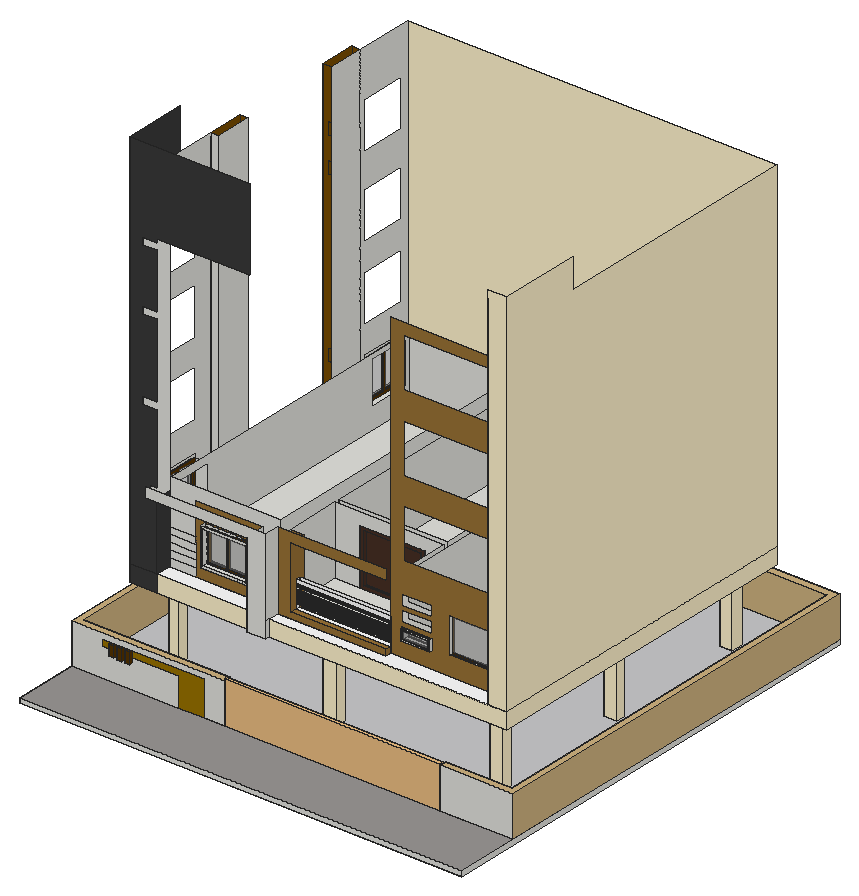
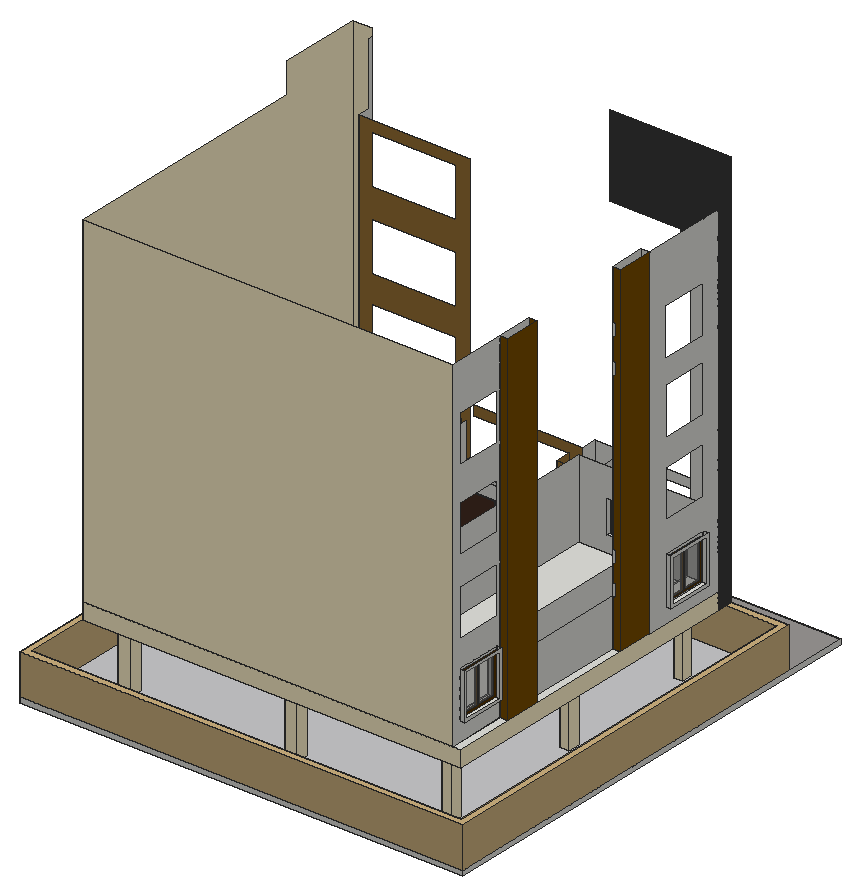
# SketchUp Ruby script. Lengths in inches.
U = 1.inch
M = Sketchup.active_model
def pt(a) = Geom::Point3d.new(a.map { |v| v * U })
def face(e, loops, mat)
  f = e.add_face(loops[0].map { |a| pt(a) })
  loops[1..].each { |l| e.add_face(l.map { |a| pt(a) }).erase! }
  f.material = f.back_material = mat if mat
  f
end
# faces: each face lists its corners as indices into pts; further lists are holes
def faces(e, pts, list, mat = nil) = list.each { |f| face(e, (f[0].is_a?(Array) ? f : [f]).map { |l| l.map { |i| pts[i] } }, mat) }
# xy, xz, yz: faces in a plane at the given z, y or x. An outline is a flat list of corners, or four numbers for a rectangle; further outlines are holes
def ring(l) = l.size == 4 ? [[l[0], l[1]], [l[2], l[1]], [l[2], l[3]], [l[0], l[3]]] : l.each_slice(2).to_a
def flat(e, list, mat, &to3) = list.each { |f| face(e, (f[0].is_a?(Array) ? f : [f]).map { |l| ring(l).map { |u, v| to3.(u, v) } }, mat) }
def xy(e, z, list, mat = nil) = flat(e, list, mat) { |x, y| [x, y, z] }
def xz(e, y, list, mat = nil) = flat(e, list, mat) { |x, z| [x, y, z] }
def yz(e, x, list, mat = nil) = flat(e, list, mat) { |y, z| [x, y, z] }
def lines(e, pts, list) = list.each { |a, b| e.add_line(pt(pts[a]), pt(pts[b])) }
# prism: a flat outline (further loops are holes) pulled along v
def prism(e, loops, v, mat = nil)
  f = face(e, loops, mat); d = Geom::Vector3d.new(v.map { |x| x * U })
  f.pushpull(f.normal.samedirection?(d) ? d.length : -d.length)
end
def box(e, o, s, mat = nil) = prism(e, [[o, [o[0] + s[0], o[1], o[2]], [o[0] + s[0], o[1] + s[1], o[2]], [o[0], o[1] + s[1], o[2]]]], [0, 0, s[2]], mat)
def at(x, y, z, deg = 0) = Geom::Transformation.translation(pt([x, y, z])) * Geom::Transformation.rotation(ORIGIN, Z_AXIS, deg.degrees)
def axes(o, x, y, z) = Geom::Transformation.new([*x, 0, *y, 0, *z, 0, *pt(o).to_a, 1])
def part(name) = M.definitions.add(name)
# library, detail: a bought-in or finely detailed component or shape, given as its bounding box
def library(name, o, s) = part(name).tap { |d| box(d.entities, o, s) }
def detail(e, o, s) = box(e.add_group.entities, o, s)
def put(e, d, t, mat = nil) = e.add_instance(d, t).tap { |i| i.material = mat if mat }
def group(e, t, mat = nil) = e.add_group.tap { |g| g.transformation = t; g.material = mat if mat }.entities
root = M.entities
M.materials.add("[Color C07]").color = [120, 76, 0]
M.materials.add("[Color C08]").color = [85, 51, 0]
M.materials.add("[Color D01]").color = [255, 242, 204]
M.materials.add("[Color D07]").color = [153, 114, 54]
M.materials.add("[Color D07]1").color = [153, 114, 0]
M.materials.add("[Color D08]").color = [95, 67, 39]
M.materials.add("[Color M00]").color = [255, 255, 255]
M.materials.add("[Color M07]").color = [58, 58, 58]
M.materials.add("[Concrete Aggregate Smoke]").color = [154, 150, 148]
M.materials.add("[Polished Concrete New]").color = [200, 200, 203]
M.materials.add("[Stone Sandstone Ashlar Light]").color = [206, 178, 128]
M.materials.add("[Translucent Glass Gray]").color = [128, 128, 128]
M.materials["[Translucent Glass Gray]"].alpha = 0.5
M.materials.add("[Wood Veneer 01]").color = [71, 47, 37]
c1 = library("gate 512k",[0,0,0],[179,6.5,74.5])
c2 = part("Group\#2")
xy(c2.entities,0,[[0,0,105.3125,8.625]],"[Wood Veneer 01]")
xy(c2.entities,6.5,[[6.5,0,98.81,8.625]],"[Wood Veneer 01]")
xy(c2.entities,132.37,[[6.5,0,98.81,8.625]],"[Wood Veneer 01]")
xy(c2.entities,138.875,[[0,0,105.3125,8.625]],"[Wood Veneer 01]")
xz(c2.entities,0,[[[0,0,105.3125,138.875],[6.5,6.5,98.81,132.37]]],"[Wood Veneer 01]")
xz(c2.entities,8.625,[[[0,0,105.3125,138.875],[6.5,6.5,98.81,132.37]],[6.5,6.5,98.81,132.37]],"[Wood Veneer 01]")
yz(c2.entities,0,[[0,0,8.625,138.875]],"[Wood Veneer 01]")
yz(c2.entities,6.5,[[0,6.5,8.625,132.37]],"[Wood Veneer 01]")
yz(c2.entities,98.81,[[0,6.5,8.625,132.37]],"[Wood Veneer 01]")
yz(c2.entities,105.3125,[[0,0,8.625,138.875]],"[Wood Veneer 01]")
c3 = part("Group\#4")
xy(c3.entities,0,[[0,0,0.4375,8.25]],"[Color C08]")
xy(c3.entities,9.875,[[0,0,0.4375,8.25]],"[Color C08]")
xz(c3.entities,0,[[0,0,0.4375,9.875]],"[Color C08]")
xz(c3.entities,0.45,[[0,0.45,0.4375,9.42]],"[Color C08]")
xz(c3.entities,4.05,[[0,0.49,0.4375,9.45]],"[Color C08]")
xz(c3.entities,4.38,[[0,0.49,0.4375,9.45]],"[Color C08]")
xz(c3.entities,7.8,[[0,0.45,0.4375,9.42]],"[Color C08]")
xz(c3.entities,8.25,[[0,0,0.4375,9.875]],"[Color C08]")
yz(c3.entities,0,[[[0,0,8.25,9.875],[0.45,0.45,4.05,0.49,4.05,9.45,0.45,9.42],[7.8,0.45,7.8,9.42,4.38,9.45,4.38,0.49]]],"[Color C08]")
yz(c3.entities,0,[[0.45,0.45,0.45,9.42,4.05,9.45,4.05,0.49],[7.8,0.45,4.38,0.49,4.38,9.45,7.8,9.42]],"[Translucent Glass Gray]")
yz(c3.entities,0.4375,[[[0,0,8.25,9.875],[0.45,0.45,0.45,9.42,4.05,9.45,4.05,0.49],[7.8,0.45,4.38,0.49,4.38,9.45,7.8,9.42]]],"[Color C08]")
p = [[0,4.05,0.49],[0,0.45,0.45],[0.4375,0.45,0.45],[0.4375,4.05,0.49],[0,7.8,0.45],[0,4.38,0.49],
  [0.4375,4.38,0.49],[0.4375,7.8,0.45],[0,0.45,9.42],[0,4.05,9.45],[0.4375,4.05,9.45],[0.4375,0.45,9.42],
  [0,4.38,9.45],[0,7.8,9.42],[0.4375,7.8,9.42],[0.4375,4.38,9.45]]
faces(c3.entities,p,[[0,1,2,3],[4,5,6,7],[8,9,10,11],[12,13,14,15]],"[Color C08]")
c4 = part("Group\#3")
xy(c4.entities,0,[[0,0,69.125,3.25]],"[Color C08]")
xy(c4.entities,1.72,[[1.72,0,67.41,3.25]],"[Color C08]")
xy(c4.entities,48.28,[[1.72,0,67.41,3.25]],"[Color C08]")
xy(c4.entities,50,[[0,0,69.125,3.25]],"[Color C08]")
xz(c4.entities,0,[[[0,0,69.125,50],[1.72,1.72,67.41,48.28]]],"[Color C08]")
xz(c4.entities,0,[[1.72,1.72,67.41,48.28]],"[Translucent Glass Gray]")
xz(c4.entities,3.25,[[[0,0,69.125,50],[1.72,1.72,67.41,48.28]]],"[Color C08]")
yz(c4.entities,0,[[0,0,3.25,50]],"[Color C08]")
yz(c4.entities,1.72,[[0,1.72,3.25,48.28]],"[Color C08]")
yz(c4.entities,67.41,[[0,1.72,3.25,48.28]],"[Color C08]")
yz(c4.entities,69.125,[[0,0,3.25,50]],"[Color C08]")
xy(root,0,[[0,0,780,833.125]])
xy(root,9,[[0,113.125,0,833.125,780,833.125,780,113.125,650.79,113.125,650.79,125.125,768,125.125,768,821.125,12,821.125,12,125.125,270.04,125.125,270.04,113.125],[96,209.125,112.5,227.9375],[367.78,209.125,390.9375,227.9375],[661.375,209.125,684,227.9375],[96,457.125,112.5,477.92],
  [661.375,461.49,684,477.92],[96,716.3125,112.5,737.125],[368.72,716.3125,389.47,737.125],[661.375,716.3125,684,737.125]])
xy(root,9,[[0,0,780,0,780,113.125,650.79,113.125,650.79,125.125,270.04,125.125,270.04,113.125,0,113.125]],"[Concrete Aggregate Smoke]")
xy(root,9,[[[12,125.125,768,821.125],[661.375,716.3125,684,737.125],[367.78,209.125,390.9375,227.9375],[368.72,716.3125,389.47,737.125],[661.375,209.125,684,227.9375],[661.375,461.49,684,477.92],[96,716.3125,112.5,737.125],[96,457.125,112.5,477.92],[96,209.125,112.5,227.9375]]],"[Polished Concrete New]")
xy(root,50.58,[[69.4,108.8125,78.47,113.125],[83.09,108.8125,92.15,113.125],[97.09,108.8125,106.15,113.125]],"[Color C08]")
xy(root,70.7,[[69.4,108.8125,78.47,113.125],[83.09,108.8125,92.15,113.125],[97.09,108.8125,106.15,113.125]],"[Color C08]")
xy(root,81,[[0,113.125,270.04,113.125,270.04,125.125,12,125.125,12,821.125,768,821.125,768,125.125,650.79,125.125,650.79,113.125,780,113.125,780,833.125,0,833.125]],"[Stone Sandstone Ashlar Light]")
xy(root,129,[[261.34,172.6875,295.1875,180.75],[96,209.125,112.5,227.9375],[367.78,209.125,390.9375,227.9375],[661.375,209.125,684,227.9375],[96,457.125,112.5,477.92],
  [661.375,461.49,684,477.92],[96,716.3125,112.5,737.125],[368.72,716.3125,389.47,737.125],[661.375,716.3125,684,737.125]])
xy(root,129,[[48.625,180.75,715.3125,776.25]],"[Color D01]")
xy(root,158,[[75,180.75,95.94,209.375],[681.47,180.75,715.3125,209.375],[295.1875,199.5625,318.6875,227.625],[318.6875,199.5625,486.25,218.375],[48.625,209.375,48.625,360.49,63,360.49,63,776.25,715.3125,776.25,715.3125,209.375,486.25,209.375,486.25,326.375,453.52,326.375,453.52,335.375,486.25,335.375,486.25,764.25,495.25,764.25,495.25,218.375,703.3125,218.375,703.3125,764.25,75,764.25,75,218.375,286.1875,218.375,286.1875,764.25,295.1875,764.25,295.1875,335.375,337.77,335.375,337.77,326.375,295.1875,326.375,295.1875,209.375],
  [75,218.375,286.1875,764.25],[318.6875,218.375,486.25,218.375,486.25,326.375,453.52,326.375,453.52,335.375,337.77,335.375,337.77,326.375,295.1875,326.375,295.1875,227.625,318.6875,227.625],[495.25,218.375,703.3125,764.25],[295.1875,335.375,486.25,764.25],[48.625,360.49,63,423.72],
  [48.625,423.72,63,608.17],[48.625,608.17,63,671.4],[48.625,671.4,63,776.25]])
xy(root,158,[[95.94,180.75,261.34,209.375],[295.1875,180.75,295.1875,199.5625,486.25,199.5625,486.25,209.375,681.47,209.375,681.47,180.75]],"[Color M00]")
xy(root,168.375,[[318.6875,199.5625,486.25,209.375]],"[Color D07]")
xy(root,168.375,[[318.6875,209.375,486.25,218.375]],"[Color M00]")
xy(root,182.15,[[158.4,200.375,241.77,209.375]])
xy(root,185.7,[[39.625,241.8125,48.625,325.0625]])
xy(root,186.15,[[162.4,200.375,237.77,209.375],[162.4,209.375,237.77,218.375]])
xy(root,186.74,[[507.06,205.375,558.75,209.375]])
xy(root,188.74,[[509.06,205.375,556.75,209.375],[509.06,209.375,556.75,218.375]])
xy(root,189.7,[[39.625,245.8125,48.625,321.0625],[48.625,245.8125,75,321.0625]])
xy(root,191.68,[[591.14,209.375,681.47,218.375]])
xy(root,191.73,[[54,679.03,63,761.4]])
xy(root,195.73,[[54,683.03,63,757.4],[63,683.03,75,757.4]])
xy(root,203.99,[[509.06,205.375,556.75,209.375],[509.06,209.375,556.75,218.375]])
xy(root,205.99,[[507.06,205.375,558.75,209.375]])
xy(root,209.5,[[318.6875,209.375,486.25,218.375]],"[Color M00]")
xz(root,0,[[0,0,780,9]])
xz(root,108.8125,[[69.4,50.58,78.47,70.7],[83.09,50.58,92.15,70.7],[97.09,50.58,106.15,70.7]],"[Color C08]")
xz(root,113.125,[[0,9,188.59,9,188.59,58.95,106.15,58.95,106.15,50.58,97.09,50.58,97.09,58.95,92.15,58.95,92.15,50.58,83.09,50.58,83.09,58.95,78.47,58.95,78.47,50.58,69.4,50.58,69.4,58.95,53.21,58.95,53.21,70.7,235.65,70.7,235.65,9,270.04,9,270.04,81,0,81],[650.79,9,780,81]])
xz(root,113.125,[[69.4,50.58,78.47,70.7],[83.09,50.58,92.15,70.7],[97.09,50.58,106.15,70.7]],"[Color C08]")
xz(root,113.125,[[188.59,9,235.65,9,235.65,70.7,106.15,70.7,106.15,58.95,188.59,58.95],[53.21,58.95,69.4,70.7],[78.47,58.95,83.09,70.7],[92.15,58.95,97.09,70.7]],"[Color D07]1")
xz(root,125.125,[[12,9,270.04,81],[650.79,9,768,81]],"[Stone Sandstone Ashlar Light]")
xz(root,172.6875,[[261.34,129,295.1875,129,295.1875,295,83.63,295,83.63,278,261.34,278]])
xz(root,180.75,[[95.94,129,261.34,158],[295.1875,129,715.3125,158],[681.47,158,715.3125,814.1875]],"[Color D01]")
xz(root,180.75,[[48.625,129,95.94,158],[48.625,158,95.94,158,95.94,278,83.63,278,83.63,295,95.94,295,95.94,418.67,70.87,418.67,70.87,431.12,95.94,431.12,95.94,561.36,70.87,561.36,70.87,573.81,95.94,573.81,95.94,670.36,70.87,670.36,70.87,682.81,95.94,682.81,95.94,689,261.34,689,261.34,833,48.625,833]],"[Color M07]")
xz(root,199.5625,[[295.1875,158,486.25,158,486.25,168.375,318.6875,168.375,318.6875,278,486.25,278,486.25,295,295.1875,295]],"[Color D07]")
xz(root,200.375,[[[158.4,182.15,241.77,248.34],[162.4,186.15,237.77,244.34]]])
xz(root,205.375,[[[507.06,186.74,558.75,205.99],[509.06,188.74,556.75,203.99]]])
xz(root,209.125,[[96,9,112.5,129],[367.78,9,390.9375,129],[661.375,9,684,129]],"[Color D01]")
xz(root,209.375,[[48.625,158,95.94,689],[95.94,158,143.14,172.15],[95.94,172.15,143.14,184.34],[[158.4,182.15,241.77,248.34],[162.4,186.15,237.77,244.34]],[95.94,184.34,143.14,196.52],
  [[507.06,186.74,558.75,205.99],[509.06,188.74,556.75,203.99]],[95.94,196.52,143.14,208.71],[95.94,208.71,143.14,220.9]])
xz(root,209.375,[[[143.14,158,261.34,278],[158.4,182.15,241.77,248.34]],[[486.25,158,681.47,158,681.47,191.68,591.14,191.68,591.14,253.18,681.47,253.18,681.47,689,486.25,689],[510.53,312.03,659.59,398.84],[510.53,446.34,659.59,533.16],[510.53,583.28,659.59,670.09],[507.06,240.37,558.75,259.62],[507.06,186.74,558.75,205.99],[507.06,214.49,558.75,233.74]]],"[Color D07]")
xz(root,209.375,[[318.6875,209.5,486.25,216.375]],"[Color M00]")
xz(root,218.375,[[[75,158,286.1875,295],[162.4,186.15,237.77,244.34]],[318.6875,158,486.25,168.375],[[495.25,158,703.3125,278],[591.14,191.68,681.47,253.18],[509.06,188.74,556.75,203.99],[509.06,216.49,556.75,231.74],[509.06,242.37,556.75,257.62]]])
xz(root,218.375,[[318.6875,209.5,486.25,216.375]],"[Color M00]")
xz(root,227.625,[[295.1875,158,318.6875,278]],"[Color D07]")
xz(root,227.9375,[[96,9,112.5,129],[367.78,9,390.9375,129],[661.375,9,684,129]],"[Color D01]")
xz(root,241.8125,[[39.625,185.7,48.625,268.95]])
xz(root,245.8125,[[39.625,189.7,48.625,264.95],[48.625,189.7,75,264.95]])
xz(root,321.0625,[[39.625,189.7,48.625,264.95],[48.625,189.7,75,264.95]])
xz(root,325.0625,[[39.625,185.7,48.625,268.95]])
xz(root,326.375,[[295.1875,158,337.77,158,337.77,256.3125,453.52,256.3125,453.52,158,486.25,158,486.25,278,295.1875,278]])
xz(root,335.375,[[295.1875,158,295.1875,278,486.25,278,486.25,158,453.52,158,453.52,256.3125,337.77,256.3125,337.77,158]])
xz(root,360.49,[[48.625,158,63,761]])
xz(root,423.72,[[48.625,158,48.625,761,63,761,63,673.33,56.4375,673.33,56.4375,651.9375,63,651.9375,63,611.45,56.4375,611.45,56.4375,590.06,63,590.06,63,315.01,56.4375,315.01,56.4375,293.62,63,293.62,63,261.95,56.4375,261.95,56.4375,240.56,63,240.56,63,158]],"[Color C07]")
xz(root,457.125,[[96,9,112.5,129]],"[Color D01]")
xz(root,461.49,[[661.375,9,684,129]],"[Color D01]")
xz(root,477.92,[[96,9,112.5,129],[661.375,9,684,129]],"[Color D01]")
xz(root,608.17,[[48.625,158,63,158,63,240.56,56.4375,240.56,56.4375,261.95,63,261.95,63,293.62,56.4375,293.62,56.4375,315.01,63,315.01,63,590.06,56.4375,590.06,56.4375,611.45,63,611.45,63,651.9375,56.4375,651.9375,56.4375,673.33,63,673.33,63,761,48.625,761]],"[Color C07]")
xz(root,671.4,[[48.625,158,63,761]],"[Color C07]")
xz(root,679.03,[[54,191.73,63,274.1]])
xz(root,683.03,[[54,195.73,63,270.1],[63,195.73,75,270.1]])
xz(root,716.3125,[[96,9,112.5,129],[368.72,9,389.47,129],[661.375,9,684,129]],"[Color D01]")
xz(root,737.125,[[96,9,112.5,129],[368.72,9,389.47,129],[661.375,9,684,129]],"[Color D01]")
xz(root,757.4,[[54,195.73,63,270.1],[63,195.73,75,270.1]])
xz(root,761.4,[[54,191.73,63,274.1]])
xz(root,764.25,[[75,158,286.1875,278],[286.1875,158,295.1875,278],[295.1875,158,486.25,278],[486.25,158,495.25,278],[495.25,158,703.3125,278]])
xz(root,776.25,[[48.625,129,715.3125,158],[63,158,715.3125,761]],"[Color D01]")
xz(root,821.125,[[12,9,768,81]],"[Stone Sandstone Ashlar Light]")
xz(root,833.125,[[0,0,780,9]])
xz(root,833.125,[[0,9,780,81]],"[Stone Sandstone Ashlar Light]")
yz(root,0,[[0,0,833.125,9]])
yz(root,0,[[113.125,9,833.125,81]],"[Stone Sandstone Ashlar Light]")
yz(root,12,[[125.125,9,821.125,81]],"[Stone Sandstone Ashlar Light]")
yz(root,39.625,[[[241.8125,185.7,325.0625,268.95],[245.8125,189.7,321.0625,264.95]]])
yz(root,48.625,[[[209.375,158,360.49,761],[242.5625,577.63,325.8125,660.88],[241.8125,452.07,325.0625,535.32],[241.8125,322.38,325.0625,405.63],[241.8125,185.7,325.0625,268.95]],[[241.8125,185.7,325.0625,268.95],[245.8125,189.7,321.0625,264.95]]])
yz(root,48.625,[[360.49,158,423.72,761],[608.17,158,671.4,761]],"[Color C07]")
yz(root,48.625,[[209.375,129,776.25,158]],"[Color D01]")
yz(root,48.625,[[180.75,129,180.75,833,291.52,833,291.52,761,209.375,761,209.375,129]],"[Color M07]")
yz(root,54,[[[679.03,191.73,761.4,274.1],[683.03,195.73,757.4,270.1]]])
yz(root,63,[[360.49,158,423.72,761],[423.72,158,608.17,240.56],[608.17,158,671.4,761],[[671.4,158,776.25,761],[679.03,595.54,761.4,677.91],[679.03,453.91,761.4,536.29],[679.03,321.73,761.4,404.1],[679.03,191.73,761.4,274.1]],[[679.03,191.73,761.4,274.1],[683.03,195.73,757.4,270.1]]])
yz(root,69.4,[[108.8125,50.58,113.125,70.7]],"[Color C08]")
yz(root,75,[[[218.375,158,764.25,278],[245.8125,189.7,321.0625,264.95],[683.03,195.73,757.4,270.1]]])
yz(root,78.47,[[108.8125,50.58,113.125,70.7]],"[Color C08]")
yz(root,83.09,[[108.8125,50.58,113.125,70.7]],"[Color C08]")
yz(root,92.15,[[108.8125,50.58,113.125,70.7]],"[Color C08]")
yz(root,95.94,[[180.75,158,209.375,278]],"[Color M07]")
yz(root,96,[[209.125,9,227.9375,129],[457.125,9,477.92,129],[716.3125,9,737.125,129]],"[Color D01]")
yz(root,97.09,[[108.8125,50.58,113.125,70.7]],"[Color C08]")
yz(root,106.15,[[108.8125,50.58,113.125,70.7]],"[Color C08]")
yz(root,112.5,[[209.125,9,227.9375,129],[457.125,9,477.92,129],[716.3125,9,737.125,129]],"[Color D01]")
yz(root,158.4,[[200.375,182.15,209.375,248.34]])
yz(root,162.4,[[200.375,186.15,209.375,244.34],[209.375,186.15,218.375,244.34]])
yz(root,237.77,[[200.375,186.15,209.375,244.34],[209.375,186.15,218.375,244.34]])
yz(root,241.77,[[200.375,182.15,209.375,248.34]])
yz(root,261.34,[[172.6875,129,172.6875,278,209.375,278,209.375,158,180.75,158,180.75,129]])
yz(root,270.04,[[113.125,9,125.125,81]],"[Stone Sandstone Ashlar Light]")
yz(root,286.1875,[[218.375,158,764.25,295]])
yz(root,295.1875,[[172.6875,129,180.75,158],[172.6875,158,199.5625,295],[199.5625,158,227.625,278],[227.625,158,326.375,278],[335.375,158,764.25,278]])
yz(root,318.6875,[[218.375,158,227.625,158,227.625,278,199.5625,278,199.5625,168.375,209.375,168.375,209.375,216.375,218.375,216.375]],"[Color D07]")
yz(root,318.6875,[[[209.375,168.375,218.375,209.5],[213.875,181.71,213.5,181.76,213.16,181.9,212.86,182.13,212.63,182.42,212.49,182.77,212.4375,183.14,212.49,183.52,212.63,183.86,212.86,184.16,213.16,184.39,213.5,184.53,213.875,184.58,214.25,184.53,214.59,184.39,214.89,184.16,215.12,183.86,215.26,183.52,215.3125,183.14,215.26,182.77,215.12,182.42,214.89,182.13,214.59,181.9,214.25,181.76],[213.875,188.08,213.5,188.13,213.16,188.27,212.86,188.5,212.63,188.8,212.49,189.15,212.4375,189.52,212.49,189.89,212.63,190.24,212.86,190.54,213.16,190.76,213.5,190.91,213.875,190.96,214.25,190.91,214.59,190.76,214.89,190.54,215.12,190.24,215.26,189.89,215.3125,189.52,215.26,189.15,215.12,188.8,214.89,188.5,214.59,188.27,214.25,188.13],[213.875,194.46,213.5,194.51,213.16,194.65,212.86,194.88,212.63,195.17,212.49,195.52,212.4375,195.89,212.49,196.27,212.63,196.61,212.86,196.91,213.16,197.14,213.5,197.28,213.875,197.33,214.25,197.28,214.59,197.14,214.89,196.91,215.12,196.61,215.26,196.27,215.3125,195.89,215.26,195.52,215.12,195.17,214.89,194.88,214.59,194.65,214.25,194.51],[213.875,201.58,213.5,201.63,213.16,201.77,212.86,202,212.63,202.3,212.49,202.65,212.4375,203.02,212.49,203.39,212.63,203.74,212.86,204.04,213.16,204.26,213.5,204.41,213.875,204.46,214.25,204.41,214.59,204.26,214.89,204.04,215.12,203.74,215.26,203.39,215.3125,203.02,215.26,202.65,215.12,202.3,214.89,202,214.59,201.77,214.25,201.63],[213.875,175.33,213.5,175.38,213.16,175.52,212.86,175.75,212.63,176.05,212.49,176.4,212.4375,176.77,212.49,177.14,212.63,177.49,212.86,177.79,213.16,178.01,213.5,178.16,213.875,178.21,214.25,178.16,214.59,178.01,214.89,177.79,215.12,177.49,215.26,177.14,215.3125,176.77,215.26,176.4,215.12,176.05,214.89,175.75,214.59,175.52,214.25,175.38]],[213.875,175.33,213.5,175.38,213.16,175.52,212.86,175.75,212.63,176.05,212.49,176.4,212.4375,176.77,212.49,177.14,212.63,177.49,212.86,177.79,213.16,178.01,213.5,178.16,213.875,178.21,214.25,178.16,214.59,178.01,214.89,177.79,215.12,177.49,215.26,177.14,215.3125,176.77,215.26,176.4,215.12,176.05,214.89,175.75,214.59,175.52,214.25,175.38],[213.875,181.71,213.5,181.76,213.16,181.9,212.86,182.13,212.63,182.42,212.49,182.77,212.4375,183.14,212.49,183.52,212.63,183.86,212.86,184.16,213.16,184.39,213.5,184.53,213.875,184.58,214.25,184.53,214.59,184.39,214.89,184.16,215.12,183.86,215.26,183.52,215.3125,183.14,215.26,182.77,215.12,182.42,214.89,182.13,214.59,181.9,214.25,181.76],[213.875,188.08,213.5,188.13,213.16,188.27,212.86,188.5,212.63,188.8,212.49,189.15,212.4375,189.52,212.49,189.89,212.63,190.24,212.86,190.54,213.16,190.76,213.5,190.91,213.875,190.96,214.25,190.91,214.59,190.76,214.89,190.54,215.12,190.24,215.26,189.89,215.3125,189.52,215.26,189.15,215.12,188.8,214.89,188.5,214.59,188.27,214.25,188.13],[213.875,194.46,213.5,194.51,213.16,194.65,212.86,194.88,212.63,195.17,212.49,195.52,212.4375,195.89,212.49,196.27,212.63,196.61,212.86,196.91,213.16,197.14,213.5,197.28,213.875,197.33,214.25,197.28,214.59,197.14,214.89,196.91,215.12,196.61,215.26,196.27,215.3125,195.89,215.26,195.52,215.12,195.17,214.89,194.88,214.59,194.65,214.25,194.51],
  [213.875,201.58,213.5,201.63,213.16,201.77,212.86,202,212.63,202.3,212.49,202.65,212.4375,203.02,212.49,203.39,212.63,203.74,212.86,204.04,213.16,204.26,213.5,204.41,213.875,204.46,214.25,204.41,214.59,204.26,214.89,204.04,215.12,203.74,215.26,203.39,215.3125,203.02,215.26,202.65,215.12,202.3,214.89,202,214.59,201.77,214.25,201.63],[209.375,209.5,218.375,216.375]],"[Color M00]")
yz(root,337.77,[[326.375,158,335.375,256.3125]])
yz(root,367.78,[[209.125,9,227.9375,129]],"[Color D01]")
yz(root,368.72,[[716.3125,9,737.125,129]],"[Color D01]")
yz(root,389.47,[[716.3125,9,737.125,129]],"[Color D01]")
yz(root,390.9375,[[209.125,9,227.9375,129]],"[Color D01]")
yz(root,453.52,[[326.375,158,335.375,256.3125]])
yz(root,486.25,[[209.375,158,218.375,168.375],[218.375,158,326.375,278],[335.375,158,764.25,278]])
yz(root,486.25,[[199.5625,158,209.375,168.375]],"[Color D07]")
yz(root,486.25,[[[209.375,168.375,218.375,209.5],[213.875,201.58,214.25,201.63,214.59,201.77,214.89,202,215.12,202.3,215.26,202.65,215.3125,203.02,215.26,203.39,215.12,203.74,214.89,204.04,214.59,204.26,214.25,204.41,213.875,204.46,213.5,204.41,213.16,204.26,212.86,204.04,212.63,203.74,212.49,203.39,212.4375,203.02,212.49,202.65,212.63,202.3,212.86,202,213.16,201.77,213.5,201.63],[213.875,194.46,214.25,194.51,214.59,194.65,214.89,194.88,215.12,195.17,215.26,195.52,215.3125,195.89,215.26,196.27,215.12,196.61,214.89,196.91,214.59,197.14,214.25,197.28,213.875,197.33,213.5,197.28,213.16,197.14,212.86,196.91,212.63,196.61,212.49,196.27,212.4375,195.89,212.49,195.52,212.63,195.17,212.86,194.88,213.16,194.65,213.5,194.51],[213.875,188.08,214.25,188.13,214.59,188.27,214.89,188.5,215.12,188.8,215.26,189.15,215.3125,189.52,215.26,189.89,215.12,190.24,214.89,190.54,214.59,190.76,214.25,190.91,213.875,190.96,213.5,190.91,213.16,190.76,212.86,190.54,212.63,190.24,212.49,189.89,212.4375,189.52,212.49,189.15,212.63,188.8,212.86,188.5,213.16,188.27,213.5,188.13],[213.875,181.71,214.25,181.76,214.59,181.9,214.89,182.13,215.12,182.42,215.26,182.77,215.3125,183.14,215.26,183.52,215.12,183.86,214.89,184.16,214.59,184.39,214.25,184.53,213.875,184.58,213.5,184.53,213.16,184.39,212.86,184.16,212.63,183.86,212.49,183.52,212.4375,183.14,212.49,182.77,212.63,182.42,212.86,182.13,213.16,181.9,213.5,181.76],[213.875,175.33,214.25,175.38,214.59,175.52,214.89,175.75,215.12,176.05,215.26,176.4,215.3125,176.77,215.26,177.14,215.12,177.49,214.89,177.79,214.59,178.01,214.25,178.16,213.875,178.21,213.5,178.16,213.16,178.01,212.86,177.79,212.63,177.49,212.49,177.14,212.4375,176.77,212.49,176.4,212.63,176.05,212.86,175.75,213.16,175.52,213.5,175.38]]],"[Color D08]")
yz(root,486.25,[[209.375,209.5,218.375,216.375]],"[Color M00]")
yz(root,495.25,[[218.375,158,764.25,278]])
yz(root,507.06,[[205.375,186.74,209.375,205.99]])
yz(root,509.06,[[205.375,188.74,209.375,203.99],[209.375,188.74,218.375,203.99]])
yz(root,556.75,[[205.375,188.74,209.375,203.99],[209.375,188.74,218.375,203.99]])
yz(root,558.75,[[205.375,186.74,209.375,205.99]])
yz(root,591.14,[[209.375,191.68,218.375,253.18]])
yz(root,650.79,[[113.125,9,125.125,81]],"[Stone Sandstone Ashlar Light]")
yz(root,661.375,[[209.125,9,227.9375,129],[461.49,9,477.92,129],[716.3125,9,737.125,129]],"[Color D01]")
yz(root,681.47,[[180.75,158,180.75,799.39,187.375,799.39,187.375,689,209.375,689,209.375,158],[209.375,191.68,218.375,253.18]])
yz(root,684,[[209.125,9,227.9375,129],[461.49,9,477.92,129],[716.3125,9,737.125,129]],"[Color D01]")
yz(root,703.3125,[[218.375,158,764.25,278]])
yz(root,715.3125,[[180.75,129,776.25,158],[180.75,158,776.25,158,776.25,761,326.375,761,326.375,814.1875,180.75,814.1875]],"[Color D01]")
yz(root,768,[[125.125,9,821.125,81]],"[Stone Sandstone Ashlar Light]")
yz(root,780,[[0,0,833.125,9]])
yz(root,780,[[113.125,9,833.125,81]],"[Stone Sandstone Ashlar Light]")
p = [[318.6875,213.5,175.38],[318.6875,213.875,175.33],[486.25,213.875,175.33],[486.25,213.5,175.38],[318.6875,214.25,175.38],[486.25,214.25,175.38],
  [318.6875,213.16,175.52],[486.25,213.16,175.52],[318.6875,214.59,175.52],[486.25,214.59,175.52],[318.6875,212.86,175.75],[486.25,212.86,175.75],
  [318.6875,214.89,175.75],[486.25,214.89,175.75],[318.6875,212.63,176.05],[486.25,212.63,176.05],[318.6875,215.12,176.05],[486.25,215.12,176.05],
  [318.6875,212.49,176.4],[486.25,212.49,176.4],[318.6875,215.26,176.4],[486.25,215.26,176.4],[318.6875,212.4375,176.77],[486.25,212.4375,176.77],
  [318.6875,215.3125,176.77],[486.25,215.3125,176.77],[318.6875,212.49,177.14],[486.25,212.49,177.14],[318.6875,215.26,177.14],[486.25,215.26,177.14],
  [318.6875,212.63,177.49],[486.25,212.63,177.49],[318.6875,215.12,177.49],[486.25,215.12,177.49],[318.6875,212.86,177.79],[486.25,212.86,177.79],
  [318.6875,214.89,177.79],[486.25,214.89,177.79],[318.6875,213.16,178.01],[486.25,213.16,178.01],[318.6875,214.59,178.01],[486.25,214.59,178.01],
  [318.6875,213.5,178.16],[486.25,213.5,178.16],[318.6875,214.25,178.16],[486.25,214.25,178.16],[318.6875,213.875,178.21],[486.25,213.875,178.21],
  [318.6875,213.5,181.76],[318.6875,213.875,181.71],[486.25,213.875,181.71],[486.25,213.5,181.76],[318.6875,214.25,181.76],[486.25,214.25,181.76],
  [318.6875,213.16,181.9],[486.25,213.16,181.9],[318.6875,214.59,181.9],[486.25,214.59,181.9],[318.6875,212.86,182.13],[486.25,212.86,182.13],
  [318.6875,214.89,182.13],[486.25,214.89,182.13],[318.6875,212.63,182.42],[486.25,212.63,182.42],[318.6875,215.12,182.42],[486.25,215.12,182.42],
  [318.6875,212.49,182.77],[486.25,212.49,182.77],[318.6875,215.26,182.77],[486.25,215.26,182.77],[318.6875,212.4375,183.14],[486.25,212.4375,183.14],
  [318.6875,215.3125,183.14],[486.25,215.3125,183.14],[318.6875,212.49,183.52],[486.25,212.49,183.52],[318.6875,215.26,183.52],[486.25,215.26,183.52],
  [318.6875,212.63,183.86],[486.25,212.63,183.86],[318.6875,215.12,183.86],[486.25,215.12,183.86],[318.6875,212.86,184.16],[486.25,212.86,184.16],
  [318.6875,214.89,184.16],[486.25,214.89,184.16],[318.6875,213.16,184.39],[486.25,213.16,184.39],[318.6875,214.59,184.39],[486.25,214.59,184.39],
  [318.6875,213.5,184.53],[486.25,213.5,184.53],[318.6875,214.25,184.53],[486.25,214.25,184.53],[318.6875,213.875,184.58],[486.25,213.875,184.58],
  [318.6875,213.16,188.27],[318.6875,213.5,188.13],[486.25,213.5,188.13],[486.25,213.16,188.27],[318.6875,213.875,188.08],[486.25,213.875,188.08],
  [318.6875,214.25,188.13],[486.25,214.25,188.13],[318.6875,214.59,188.27],[486.25,214.59,188.27],[318.6875,212.86,188.5],[486.25,212.86,188.5],
  [318.6875,214.89,188.5],[486.25,214.89,188.5],[318.6875,212.63,188.8],[486.25,212.63,188.8],[318.6875,215.12,188.8],[486.25,215.12,188.8],
  [318.6875,212.49,189.15],[486.25,212.49,189.15],[318.6875,215.26,189.15],[486.25,215.26,189.15],[318.6875,212.4375,189.52],[486.25,212.4375,189.52],
  [318.6875,215.3125,189.52],[486.25,215.3125,189.52],[318.6875,212.49,189.89],[486.25,212.49,189.89],[318.6875,215.26,189.89],[486.25,215.26,189.89],
  [318.6875,212.63,190.24],[486.25,212.63,190.24],[318.6875,215.12,190.24],[486.25,215.12,190.24],[318.6875,212.86,190.54],[486.25,212.86,190.54],
  [318.6875,214.89,190.54],[486.25,214.89,190.54],[318.6875,213.16,190.76],[486.25,213.16,190.76],[318.6875,214.59,190.76],[486.25,214.59,190.76],
  [318.6875,213.5,190.91],[486.25,213.5,190.91],[318.6875,214.25,190.91],[486.25,214.25,190.91],[318.6875,213.875,190.96],[486.25,213.875,190.96],
  [318.6875,213.16,194.65],[318.6875,213.5,194.51],[486.25,213.5,194.51],[486.25,213.16,194.65],[318.6875,213.875,194.46],[486.25,213.875,194.46],
  [318.6875,214.25,194.51],[486.25,214.25,194.51],[318.6875,214.59,194.65],[486.25,214.59,194.65],[318.6875,212.86,194.88],[486.25,212.86,194.88],
  [318.6875,214.89,194.88],[486.25,214.89,194.88],[318.6875,212.63,195.17],[486.25,212.63,195.17],[318.6875,215.12,195.17],[486.25,215.12,195.17],
  [318.6875,212.49,195.52],[486.25,212.49,195.52],[318.6875,215.26,195.52],[486.25,215.26,195.52],[318.6875,212.4375,195.89],[486.25,212.4375,195.89],
  [318.6875,215.3125,195.89],[486.25,215.3125,195.89],[318.6875,212.49,196.27],[486.25,212.49,196.27],[318.6875,215.26,196.27],[486.25,215.26,196.27],
  [318.6875,212.63,196.61],[486.25,212.63,196.61],[318.6875,215.12,196.61],[486.25,215.12,196.61],[318.6875,212.86,196.91],[486.25,212.86,196.91],
  [318.6875,214.89,196.91],[486.25,214.89,196.91],[318.6875,213.16,197.14],[486.25,213.16,197.14],[318.6875,214.59,197.14],[486.25,214.59,197.14],
  [318.6875,213.5,197.28],[486.25,213.5,197.28],[318.6875,214.25,197.28],[486.25,214.25,197.28],[318.6875,213.875,197.33],[486.25,213.875,197.33],
  [318.6875,213.16,201.77],[318.6875,213.5,201.63],[486.25,213.5,201.63],[486.25,213.16,201.77],[318.6875,213.875,201.58],[486.25,213.875,201.58],
  [318.6875,214.25,201.63],[486.25,214.25,201.63],[318.6875,214.59,201.77],[486.25,214.59,201.77],[318.6875,212.86,202],[486.25,212.86,202],
  [318.6875,214.89,202],[486.25,214.89,202],[318.6875,212.63,202.3],[486.25,212.63,202.3],[318.6875,215.12,202.3],[486.25,215.12,202.3],
  [318.6875,212.49,202.65],[486.25,212.49,202.65],[318.6875,215.26,202.65],[486.25,215.26,202.65],[318.6875,212.4375,203.02],[486.25,212.4375,203.02],
  [318.6875,215.3125,203.02],[486.25,215.3125,203.02],[318.6875,212.49,203.39],[486.25,212.49,203.39],[318.6875,215.26,203.39],[486.25,215.26,203.39],
  [318.6875,212.63,203.74],[486.25,212.63,203.74],[318.6875,215.12,203.74],[486.25,215.12,203.74],[318.6875,212.86,204.04],[486.25,212.86,204.04],
  [318.6875,214.89,204.04],[486.25,214.89,204.04],[318.6875,213.16,204.26],[486.25,213.16,204.26],[318.6875,214.59,204.26],[486.25,214.59,204.26],
  [318.6875,213.5,204.41],[486.25,213.5,204.41],[318.6875,214.25,204.41],[486.25,214.25,204.41],[318.6875,213.875,204.46],[486.25,213.875,204.46]]
faces(root,p,[[0,1,2,3],[1,4,5,2],[6,0,3,7],[4,8,9,5],[10,6,7,11],[8,12,13,9],[14,10,11,15],[12,16,17,13],
  [18,14,15,19],[16,20,21,17],[22,18,19,23],[20,24,25,21],[26,22,23,27],[24,28,29,25],[30,26,27,31],[28,32,33,29],
  [34,30,31,35],[32,36,37,33],[38,34,35,39],[36,40,41,37],[42,38,39,43],[40,44,45,41],[46,42,43,47],[44,46,47,45],
  [48,49,50,51],[49,52,53,50],[54,48,51,55],[52,56,57,53],[58,54,55,59],[56,60,61,57],[62,58,59,63],[60,64,65,61],
  [66,62,63,67],[64,68,69,65],[70,66,67,71],[68,72,73,69],[74,70,71,75],[72,76,77,73],[78,74,75,79],[76,80,81,77],
  [82,78,79,83],[80,84,85,81],[86,82,83,87],[84,88,89,85],[90,86,87,91],[88,92,93,89],[94,90,91,95],[92,94,95,93],
  [96,97,98,99],[97,100,101,98],[100,102,103,101],[102,104,105,103],[106,96,99,107],[104,108,109,105],[110,106,107,111],[108,112,113,109],
  [114,110,111,115],[112,116,117,113],[118,114,115,119],[116,120,121,117],[122,118,119,123],[120,124,125,121],[126,122,123,127],[124,128,129,125],
  [130,126,127,131],[128,132,133,129],[134,130,131,135],[132,136,137,133],[138,134,135,139],[136,140,141,137],[142,138,139,143],[140,142,143,141],
  [144,145,146,147],[145,148,149,146],[148,150,151,149],[150,152,153,151],[154,144,147,155],[152,156,157,153],[158,154,155,159],[156,160,161,157],
  [162,158,159,163],[160,164,165,161],[166,162,163,167],[164,168,169,165],[170,166,167,171],[168,172,173,169],[174,170,171,175],[172,176,177,173],
  [178,174,175,179],[176,180,181,177],[182,178,179,183],[180,184,185,181],[186,182,183,187],[184,188,189,185],[190,186,187,191],[188,190,191,189],
  [192,193,194,195],[193,196,197,194],[196,198,199,197],[198,200,201,199],[202,192,195,203],[200,204,205,201],[206,202,203,207],[204,208,209,205],
  [210,206,207,211],[208,212,213,209],[214,210,211,215],[212,216,217,213],[218,214,215,219],[216,220,221,217],[222,218,219,223],[220,224,225,221],
  [226,222,223,227],[224,228,229,225],[230,226,227,231],[228,232,233,229],[234,230,231,235],[232,236,237,233],[238,234,235,239],[236,238,239,237]],"[Color M00]")
put(root,c1,axes([650.79,113.125,9],[-2.12707,0,0],[0,1,0],[0,0,1]))
put(root,c2,axes([337.77,326.375,158],[1.09911,0,0],[0,0.6,0],[0,0,0.70792]))
put(root,c3,axes([237.77,209.375,186.15],[0,6.04632,0],[-9.13636,0,0],[0,0,5.89241]))
put(root,c4,axes([509.06,206,188.74],[0.68987,0,0],[0,0.35,0],[0,0,0.305]))
put(root,c3,axes([48.625,245.8125,189.7],[8.6376,0,0],[0,9.1053,0],[0,0,7.62025]))
put(root,c4,axes([591.14,212.66,191.68],[1.30671,0,0],[0,1,0],[0,0,1.23007]))
put(root,c3,axes([62.14,683.03,195.73],[8.6376,0,0],[0,9.01515,0],[0,0,7.53165]))
